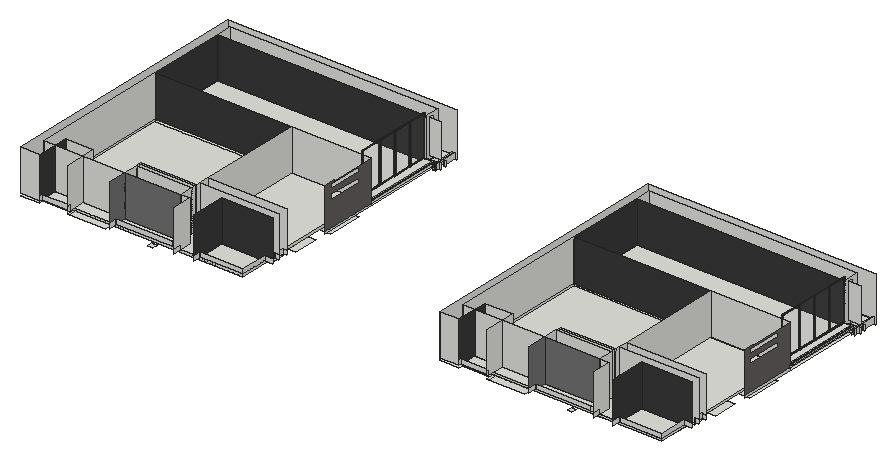
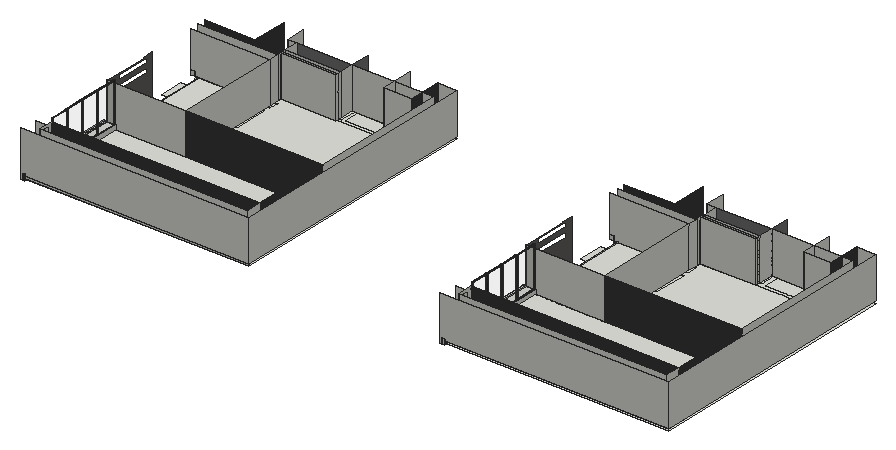
# SketchUp Ruby script. Lengths in inches.
U = 1.inch
M = Sketchup.active_model
def pt(a) = Geom::Point3d.new(a.map { |v| v * U })
def face(e, loops, mat)
  f = e.add_face(loops[0].map { |a| pt(a) })
  loops[1..].each { |l| e.add_face(l.map { |a| pt(a) }).erase! }
  f.material = f.back_material = mat if mat
  f
end
# faces: each face lists its corners as indices into pts; further lists are holes
def faces(e, pts, list, mat = nil) = list.each { |f| face(e, (f[0].is_a?(Array) ? f : [f]).map { |l| l.map { |i| pts[i] } }, mat) }
# xy, xz, yz: faces in a plane at the given z, y or x. An outline is a flat list of corners, or four numbers for a rectangle; further outlines are holes
def ring(l) = l.size == 4 ? [[l[0], l[1]], [l[2], l[1]], [l[2], l[3]], [l[0], l[3]]] : l.each_slice(2).to_a
def flat(e, list, mat, &to3) = list.each { |f| face(e, (f[0].is_a?(Array) ? f : [f]).map { |l| ring(l).map { |u, v| to3.(u, v) } }, mat) }
def xy(e, z, list, mat = nil) = flat(e, list, mat) { |x, y| [x, y, z] }
def xz(e, y, list, mat = nil) = flat(e, list, mat) { |x, z| [x, y, z] }
def yz(e, x, list, mat = nil) = flat(e, list, mat) { |y, z| [x, y, z] }
def lines(e, pts, list) = list.each { |a, b| e.add_line(pt(pts[a]), pt(pts[b])) }
# prism: a flat outline (further loops are holes) pulled along v
def prism(e, loops, v, mat = nil)
  f = face(e, loops, mat); d = Geom::Vector3d.new(v.map { |x| x * U })
  f.pushpull(f.normal.samedirection?(d) ? d.length : -d.length)
end
def box(e, o, s, mat = nil) = prism(e, [[o, [o[0] + s[0], o[1], o[2]], [o[0] + s[0], o[1] + s[1], o[2]], [o[0], o[1] + s[1], o[2]]]], [0, 0, s[2]], mat)
def at(x, y, z, deg = 0) = Geom::Transformation.translation(pt([x, y, z])) * Geom::Transformation.rotation(ORIGIN, Z_AXIS, deg.degrees)
def axes(o, x, y, z) = Geom::Transformation.new([*x, 0, *y, 0, *z, 0, *pt(o).to_a, 1])
def part(name) = M.definitions.add(name)
# library, detail: a bought-in or finely detailed component or shape, given as its bounding box
def library(name, o, s) = part(name).tap { |d| box(d.entities, o, s) }
def detail(e, o, s) = box(e.add_group.entities, o, s)
def put(e, d, t, mat = nil) = e.add_instance(d, t).tap { |i| i.material = mat if mat }
def group(e, t, mat = nil) = e.add_group.tap { |g| g.transformation = t; g.material = mat if mat }.entities
root = M.entities
M.materials.add("Glazing").color = [128, 128, 128]
M.materials["Glazing"].alpha = 0.05
M.materials.add("Powdercoating").color = [41, 44, 40]
M.materials.add("[Color M05]").color = [114, 114, 114]
M.materials.add("[Color M07]").color = [58, 58, 58]
M.materials.add("[Concrete Tile]").color = [165, 155, 133]
M.materials.add("[Stone Marble]").color = [99, 95, 94]
c1 = part("Group\#15")
xy(c1.entities,0,[[0,-55.94,0.71,45.94]])
xy(c1.entities,0.2,[[0,-55.94,0.47,45.94],[0.47,45.94,0.71,46.42]])
xy(c1.entities,2.36,[[0.47,-55.94,0.71,46.42]])
xz(c1.entities,-55.94,[[0,0,0.71,0,0.71,2.36,0.47,2.36,0.47,0.2,0,0.2]])
xz(c1.entities,45.94,[[0,0,0.71,0.2]])
xz(c1.entities,46.42,[[0.47,0.2,0.71,2.36]])
yz(c1.entities,0,[[-55.94,0,45.94,0.2]])
yz(c1.entities,0.47,[[-55.94,0.2,46.42,2.36]])
yz(c1.entities,0.71,[[-55.94,0,45.94,0,45.94,0.2,46.42,0.2,46.42,2.36,-55.94,2.36]])
c2 = part("Group\#7")
xy(c2.entities,0,[[0,-59.09,0.71,45.94]])
xy(c2.entities,0.2,[[0,-59.09,0.47,45.94],[0.47,45.94,0.71,46.42]])
xy(c2.entities,2.36,[[0.47,-59.09,0.71,46.42]])
xz(c2.entities,-59.09,[[0,0,0.71,0,0.71,2.36,0.47,2.36,0.47,0.2,0,0.2]])
xz(c2.entities,45.94,[[0,0,0.71,0.2]])
xz(c2.entities,46.42,[[0.47,0.2,0.71,2.36]])
yz(c2.entities,0,[[-59.09,0,45.94,0.2]])
yz(c2.entities,0.47,[[-59.09,0.2,46.42,2.36]])
yz(c2.entities,0.71,[[-59.09,0,45.94,0,45.94,0.2,46.42,0.2,46.42,2.36,-59.09,2.36]])
c3 = part("Group\#16")
prism(c3.entities,[[[0.47,-56.18,0.2],[0,-56.18,0.2],[0,-56.18,0],[0.71,-56.18,0],[0.71,-56.18,2.36],[0.47,-56.18,2.36]]],[0,28.68,0])
c4 = part("Group\#10")
box(c4.entities,[-0.73,0,0],[27.99,0.55,102.05])
c5 = part("Group\#18")
xy(c5.entities,0,[[0.47,-56.18,0.47,-55.47,0,-55.47,0,-28.21,1.18,-28.21,1.18,-56.18]])
xy(c5.entities,0.2,[[0.71,-56.18,1.18,-28.21],[0,-55.47,0.47,-28.21],[0.47,-28.21,0.71,-27.74]])
xy(c5.entities,2.36,[[0.47,-56.18,0.71,-27.74]])
xz(c5.entities,-56.18,[[0.47,0,1.18,0,1.18,0.2,0.71,0.2,0.71,2.36,0.47,2.36]])
xz(c5.entities,-55.47,[[0,0,0.47,0.2]])
xz(c5.entities,-28.21,[[0,0,1.18,0.2]])
xz(c5.entities,-27.74,[[0.47,0.2,0.71,2.36]])
yz(c5.entities,0,[[-55.47,0,-28.21,0.2]])
yz(c5.entities,0.47,[[-56.18,0,-55.47,0.2],[-56.18,0.2,-27.74,2.36]])
yz(c5.entities,0.71,[[-56.18,0.2,-27.74,2.36]])
yz(c5.entities,1.18,[[-56.18,0,-28.21,0.2]])
c6 = part("Group\#34")
xy(c6.entities,0,[[-20.45,0,7.76,1.22]])
xy(c6.entities,0.06,[[-20.39,0.06,7.7,1.22]])
xy(c6.entities,0.47,[[-19.98,0,7.28,0.06]])
xy(c6.entities,101.89,[[-19.98,0,7.28,0.06]])
xy(c6.entities,102.3,[[-20.39,0.06,7.7,1.22]])
xy(c6.entities,102.36,[[-20.45,0,7.76,1.22]])
xz(c6.entities,0,[[[-20.45,0,7.76,102.36],[-19.98,0.47,7.28,101.89]]])
xz(c6.entities,0.06,[[[-20.39,0.06,7.7,102.3],[-19.98,0.47,7.28,101.89]]])
xz(c6.entities,1.22,[[[-20.45,0,7.76,102.36],[-20.39,0.06,7.7,102.3]]])
yz(c6.entities,-20.45,[[0,0,1.22,102.36]])
yz(c6.entities,-20.39,[[0.06,0.06,1.22,102.3]])
yz(c6.entities,-19.98,[[0,0.47,0.06,101.89]])
yz(c6.entities,7.28,[[0,0.47,0.06,101.89]])
yz(c6.entities,7.7,[[0.06,0.06,1.22,102.3]])
yz(c6.entities,7.76,[[0,0,1.22,102.36]])
c7 = part("Group\#6")
put(c7.entities,c1,axes([27.97,0,7.875],[1,0,0],[0,0,-1],[0,1,0]),"Powdercoating")
put(c7.entities,c2,axes([0.71,0,6.8],[-1,0,0],[0,0,-0.97687],[0,1,0]),"Powdercoating")
put(c7.entities,c3,axes([-27.5,0,-38.07],[0,0,-1],[-1,0,0],[0,1,0]),"Powdercoating")
put(c7.entities,c4,at(1.12,0.35,-38.39),"Glazing")
put(c7.entities,c5,axes([-27.5,0,63.35],[0,0,1],[-1,0,0],[0,1,0]),"Powdercoating")
put(c7.entities,c6,at(20.6875,1.0625,-38.54),"Powdercoating")
c8 = part("Sliding door assembly")
put(c8.entities,c7,at(-1.18,4.5,38.86))
g1 = group(c8.entities,at(84.74,4.5,38.86))
put(g1,c1,axes([-27.97,0,7.875],[-1,0,0],[0,0,-1],[0,1,0]),"Powdercoating")
put(g1,c2,axes([-0.71,0,6.8],[1,0,0],[0,0,-0.97687],[0,1,0]),"Powdercoating")
put(g1,c3,axes([27.5,0,-38.07],[0,0,-1],[1,0,0],[0,1,0]),"Powdercoating")
put(g1,c4,axes([-1.12,0.35,-38.39],[-1,0,0],[0,1,0],[0,0,1]),"Glazing")
put(g1,c5,axes([27.5,0,63.35],[0,0,1],[1,0,0],[0,1,0]),"Powdercoating")
put(g1,c6,axes([-20.6875,1.0625,-38.54],[-1,0,0],[0,1,0],[0,0,1]),"Powdercoating")
g2 = group(c8.entities,at(56.0625,4.5,38.86))
put(g2,c1,axes([-27.97,0,7.875],[-1,0,0],[0,0,-1],[0,1,0]),"Powdercoating")
put(g2,c3,axes([27.5,0,-38.07],[0,0,-1],[1,0,0],[0,1,0]),"Powdercoating")
put(g2,c4,axes([-1.12,0.35,-38.39],[-1,0,0],[0,1,0],[0,0,1]),"Glazing")
put(g2,c5,axes([27.5,0,63.35],[0,0,1],[1,0,0],[0,1,0]),"Powdercoating")
put(g2,c6,axes([-20.6875,1.0625,-38.54],[-1,0,0],[0,1,0],[0,0,1]),"Powdercoating")
g3 = group(g2,at(-0.71,0,6.8),"Powdercoating")
xy(g3,-45.34,[[0.47,0.2,0.71,2.36]])
xy(g3,-44.88,[[0,0,0.71,0.2]])
xy(g3,57.73,[[0,0,0.71,0,0.71,2.36,0.47,2.36,0.47,0.2,0,0.2]])
xz(g3,0,[[0,-44.88,0.71,57.73]])
xz(g3,0.2,[[0.47,-45.34,0.71,-44.88],[0,-44.88,0.47,57.73]])
xz(g3,2.36,[[0.47,-45.34,0.71,57.73]])
yz(g3,0,[[0,-44.88,0.2,57.73]])
yz(g3,0.47,[[0.2,-45.34,2.36,57.73]])
yz(g3,0.71,[[0.2,-45.34,2.36,-45.34,2.36,57.73,0,57.73,0,-44.88,0.2,-44.88]])
put(c8.entities,c7,axes([-33.94,4.5,38.86],[1.14218,0,0],[0,1,0],[0,0,1]))
c9 = part("sliding door")
put(c9.entities,c8,at(0,-4.5,-0.08))
xy(root,117.41,[[671.25,2113.57,913.875,2213.62],[1889.4375,2113.57,2132.0625,2213.62]])
xy(root,126,[[262.875,1799.9375,262.875,2554.375,913.875,2554.375,913.875,2483.21,890.875,2483.21,890.875,2531.375,285.875,2531.375,285.875,1822.9375,319.53,1822.9375,319.53,1799.9375],[399.88,1799.9375,406.68,1822.9375],[406.68,1799.9375,511.23,1822.9375],[634.11,1799.9375,647.8,1814.92],[1481.0625,1799.9375,1481.0625,2554.375,2132.0625,2554.375,2132.0625,2483.21,2109.0625,2483.21,2109.0625,2531.375,1504.0625,2531.375,1504.0625,1822.9375,1537.72,1822.9375,1537.72,1799.9375],
  [1618.07,1799.9375,1624.87,1822.9375],[1624.87,1799.9375,1729.42,1822.9375],[1852.3,1799.9375,1865.99,1814.92],[319.53,1811.4375,399.88,1822.9375],[1537.72,1811.4375,1618.07,1822.9375],
  [285.875,1822.9375,319.53,1834.0625],[319.53,1822.9375,399.88,1834.0625],[399.88,1822.9375,406.68,1834.0625],[406.68,1822.9375,511.23,1834.0625],[511.23,1822.9375,521.59,1834.0625],
  [521.59,1822.9375,634.11,1834.0625],[634.11,1822.9375,709.87,1834.0625],[709.87,1822.9375,767.19,1834.0625],[767.19,1822.9375,817,1834.0625],[817,1822.9375,890.875,1834.0625],
  [1504.0625,1822.9375,1537.72,1834.0625],[1537.72,1822.9375,1618.07,1834.0625],[1618.07,1822.9375,1624.87,1834.0625],[1624.87,1822.9375,1729.42,1834.0625],[1729.42,1822.9375,1739.78,1834.0625],
  [1739.78,1822.9375,1852.3,1834.0625],[1852.3,1822.9375,1928.05,1834.0625],[1928.05,1822.9375,1985.38,1834.0625],[1985.38,1822.9375,2035.1875,1834.0625],[2035.1875,1822.9375,2109.0625,1834.0625],
  [285.875,1834.0625,319.53,1834.0625,319.53,1893.25,399.88,1893.25,399.88,1834.0625,406.68,1834.0625,406.68,1893.25,511.23,1893.25,511.23,1834.0625,521.59,1834.0625,521.59,1893.25,709.87,1893.25,709.87,1834.0625,767.19,1834.0625,767.19,1902.66,285.875,1902.66],[319.53,1834.0625,399.88,1893.25],[406.68,1834.0625,511.23,1893.25],[521.59,1834.0625,634.11,1893.25],[634.11,1834.0625,709.87,1893.25],
  [767.19,1834.0625,817,1902.66],[817,1834.0625,890.875,1902.66],[1504.0625,1834.0625,1537.72,1834.0625,1537.72,1893.25,1618.07,1893.25,1618.07,1834.0625,1624.87,1834.0625,1624.87,1893.25,1729.42,1893.25,1729.42,1834.0625,1739.78,1834.0625,1739.78,1893.25,1928.05,1893.25,1928.05,1834.0625,1985.38,1834.0625,1985.38,1902.66,1504.0625,1902.66],[1537.72,1834.0625,1618.07,1893.25],[1624.87,1834.0625,1729.42,1893.25],
  [1739.78,1834.0625,1852.3,1893.25],[1852.3,1834.0625,1928.05,1893.25],[1985.38,1834.0625,2035.1875,1902.66],[2035.1875,1834.0625,2109.0625,1902.66],[285.875,1902.66,817,1902.66,817,1926.07,683.6875,1926.07,683.6875,1953.7,817,1953.7,817,1970.91,683.6875,1970.91,683.6875,2070.28,890.875,2070.28,890.875,2257.8125,285.875,2257.8125],
  [817,1902.66,890.875,1926.07],[1504.0625,1902.66,2035.1875,1902.66,2035.1875,1926.07,1901.875,1926.07,1901.875,1953.7,2035.1875,1953.7,2035.1875,1970.91,1901.875,1970.91,1901.875,2070.28,2109.0625,2070.28,2109.0625,2257.8125,1504.0625,2257.8125],[2035.1875,1902.66,2109.0625,1926.07],[683.6875,1926.07,817,1953.7],[817,1926.07,890.875,1953.7],
  [890.875,1926.07,902.375,1953.7],[1901.875,1926.07,2035.1875,1953.7],[1901.875,1926.07,2035.1875,1953.7],[2035.1875,1926.07,2109.0625,1953.7],[2109.0625,1926.07,2120.5625,1953.7],
  [817,1953.7,890.875,1970.91],[2035.1875,1953.7,2109.0625,1970.91],[683.6875,1970.91,890.875,2070.28],[1901.875,1970.91,2109.0625,2070.28],[890.875,1987.85,913.875,2059.15],
  [2109.0625,1987.85,2132.0625,2059.15],[285.875,2257.8125,890.875,2485.84],[890.875,2257.8125,913.875,2483.21],[1504.0625,2257.8125,2109.0625,2485.84],[2109.0625,2257.8125,2132.0625,2483.21]])
xy(root,132,[[262.875,1799.9375,262.875,2554.375,913.875,2554.375,913.875,2483.21,890.875,2483.21,890.875,2531.375,285.875,2531.375,285.875,1822.9375,319.53,1822.9375,319.53,1799.9375],[1481.0625,1799.9375,1481.0625,2554.375,2132.0625,2554.375,2132.0625,2483.21,2109.0625,2483.21,2109.0625,2531.375,1504.0625,2531.375,1504.0625,1822.9375,1537.72,1822.9375,1537.72,1799.9375],[319.53,1807.625,399.88,1822.9375],[1537.72,1807.625,1618.07,1822.9375],[285.875,1822.9375,319.53,1855.75],
  [319.53,1822.9375,399.88,1855.75],[399.88,1822.9375,523.04,1855.75],[523.04,1822.9375,683.6875,1855.75],[683.6875,1822.9375,709.87,1855.75],[709.87,1822.9375,709.87,1855.75,683.6875,1855.75,683.6875,1926.07,890.875,1926.07,890.875,1902.66,767.19,1902.66,767.19,1822.9375],
  [767.19,1822.9375,890.875,1902.66],[1504.0625,1822.9375,1537.72,1855.75],[1537.72,1822.9375,1618.07,1855.75],[1618.07,1822.9375,1741.23,1855.75],[1741.23,1822.9375,1901.875,1855.75],
  [1901.875,1822.9375,1928.05,1855.75],[1928.05,1822.9375,1928.05,1855.75,1901.875,1855.75,1901.875,1926.07,2109.0625,1926.07,2109.0625,1902.66,1985.38,1902.66,1985.38,1822.9375],[1985.38,1822.9375,2109.0625,1902.66],[319.53,1855.75,399.88,1893.25],[523.04,1855.75,683.6875,1897.5625],
  [1537.72,1855.75,1618.07,1893.25],[1741.23,1855.75,1901.875,1897.5625],[523.04,1897.5625,683.6875,1906.6875],[1741.23,1897.5625,1901.875,1906.6875],[523.04,1906.6875,683.6875,1913.4375],
  [1741.23,1906.6875,1901.875,1913.4375],[683.6875,1926.07,890.875,1953.7],[890.875,1926.07,902.375,1953.7],[1901.875,1926.07,2109.0625,1953.7],[2109.0625,1926.07,2120.5625,1953.7],
  [683.6875,1953.7,890.875,2258.18],[1901.875,1953.7,2109.0625,2258.18],[285.875,2258.18,886.75,2258.18,886.75,2483.21,890.875,2483.21,890.875,2486.82,285.875,2486.82],[886.75,2258.18,890.875,2483.21],[890.875,2258.18,913.875,2483.21],
  [1504.0625,2258.18,2104.9375,2258.18,2104.9375,2483.21,2109.0625,2483.21,2109.0625,2486.82,1504.0625,2486.82],[2104.9375,2258.18,2109.0625,2483.21],[2109.0625,2258.18,2132.0625,2483.21]])
xy(root,143.875,[[913.875,2257.8125,921.125,2258.18],[2132.0625,2257.8125,2139.3125,2258.18],[886.75,2258.18,913.875,2483.21],[913.875,2258.18,921.125,2483.21],[2104.9375,2258.18,2132.0625,2483.21],
  [2132.0625,2258.18,2139.3125,2483.21],[913.875,2483.21,921.125,2486.82],[2132.0625,2483.21,2139.3125,2486.82]])
xy(root,144.25,[[913.875,2257.8125,921.125,2258.18],[2132.0625,2257.8125,2139.3125,2258.18]])
xz(root,1799.9375,[[262.875,132,319.53,252],[1481.0625,132,1537.72,252]])
xz(root,1799.9375,[[521.59,132,523.04,252],[1739.78,132,1741.23,252]],"[Concrete Tile]")
xz(root,1807.625,[[319.53,132,399.88,145.375],[1537.72,132,1618.07,145.375]])
xz(root,1814.92,[[634.11,124.32,647.8,126],[1852.3,124.32,1865.99,126]])
xz(root,1822.9375,[[285.875,126,890.875,132],[1504.0625,126,2109.0625,132],[523.04,132,683.6875,145.375],[683.6875,132,709.87,145.375],[767.19,132,890.875,145.375],
  [1741.23,132,1901.875,145.375],[1901.875,132,1928.05,145.375],[1985.38,132,2109.0625,145.375]])
xz(root,1855.75,[[285.875,132,523.04,252],[683.6875,132,709.87,252],[1504.0625,132,1741.23,252],[1901.875,132,1928.05,252]])
xz(root,1855.75,[[523.04,132,683.6875,252],[1741.23,132,1901.875,252]],"[Color M05]")
xz(root,1893.25,[[319.53,132,399.88,252],[1537.72,132,1618.07,252]])
xz(root,1897.5625,[[523.04,132,683.6875,252],[1741.23,132,1901.875,252]])
xz(root,1902.66,[[890.875,132,913.875,145.375],[2109.0625,132,2132.0625,145.375]])
xz(root,1902.66,[[767.19,132,890.875,132,890.875,147.125,913.875,147.125,913.875,252,767.19,252],[1985.38,132,2109.0625,132,2109.0625,147.125,2132.0625,147.125,2132.0625,252,1985.38,252]],"[Color M07]")
xz(root,1906.6875,[[523.04,132,683.6875,252],[1741.23,132,1901.875,252]])
xz(root,1913.4375,[[523.04,132,683.6875,252],[1741.23,132,1901.875,252]])
xz(root,1926.07,[[683.6875,132,683.6875,252,913.875,252,913.875,145.375,902.375,145.375,902.375,132],[902.375,132,913.875,145.375],[1901.875,132,1901.875,252,2132.0625,252,2132.0625,145.375,2120.5625,145.375,2120.5625,132],[2120.5625,132,2132.0625,145.375]])
xz(root,1953.7,[[683.6875,132,902.375,132,902.375,145.375,913.875,145.375,913.875,252,683.6875,252],[902.375,132,913.875,145.375],[1901.875,132,2120.5625,132,2120.5625,145.375,2132.0625,145.375,2132.0625,252,1901.875,252],[2120.5625,132,2132.0625,145.375]])
xz(root,2257.8125,[[913.875,143.875,921.125,144.25],[2132.0625,143.875,2139.3125,144.25]])
xz(root,2258.18,[[683.6875,132,683.6875,252,913.875,252,913.875,143.875,886.75,143.875,886.75,132],[886.75,132,913.875,143.875],[1901.875,132,1901.875,252,2132.0625,252,2132.0625,143.875,2104.9375,143.875,2104.9375,132],[2104.9375,132,2132.0625,143.875],[913.875,143.875,921.125,144.25],
  [2132.0625,143.875,2139.3125,144.25],[913.875,144.25,921.125,145.375],[2132.0625,144.25,2139.3125,145.375]])
xz(root,2258.18,[[285.875,132,683.6875,252],[1504.0625,132,1901.875,252]],"[Color M07]")
xz(root,2483.21,[[886.75,132,890.875,136.875],[2104.9375,132,2109.0625,136.875],[886.75,136.875,890.875,143.875],[2104.9375,136.875,2109.0625,143.875],[913.875,143.875,921.125,145.375],
  [2132.0625,143.875,2139.3125,145.375]])
xz(root,2483.21,[[890.875,132,913.875,136.875],[2109.0625,132,2132.0625,136.875],[890.875,136.875,913.875,143.875],[2109.0625,136.875,2132.0625,143.875]],"[Color M07]")
xz(root,2486.82,[[913.875,120.4375,921.125,136.875],[2132.0625,120.4375,2139.3125,136.875],[913.875,136.875,921.125,143.875],[2132.0625,136.875,2139.3125,143.875]])
xz(root,2486.82,[[285.875,132,890.875,252],[1504.0625,132,2109.0625,252]],"[Color M07]")
xz(root,2497.47,[[921.125,120.4375,927.0625,136.875],[2139.3125,120.4375,2145.25,136.875],[927.0625,143.875,927.0625,145.375,890.875,145.375,890.875,245.15,927.75,245.15,927.75,143.875],[2145.25,143.875,2145.25,145.375,2109.0625,145.375,2109.0625,245.15,2145.9375,245.15,2145.9375,143.875]])
xz(root,2514.84,[[921.125,120.4375,927.0625,136.875],[2139.3125,120.4375,2145.25,136.875]])
xz(root,2531.375,[[285.875,126,890.875,132],[1504.0625,126,2109.0625,132],[285.875,132,890.875,252],[1504.0625,132,2109.0625,252]])
xz(root,2554.375,[[921.125,120.4375,921.125,136.875,913.875,136.875,913.875,132,262.875,132,262.875,252,927.75,252,927.75,120.4375],[913.875,120.4375,921.125,136.875],[2139.3125,120.4375,2139.3125,136.875,2132.0625,136.875,2132.0625,132,1481.0625,132,1481.0625,252,2145.9375,252,2145.9375,120.4375],[2132.0625,120.4375,2139.3125,136.875],[1481.0625,126,2132.0625,132]])
yz(root,262.875,[[1799.9375,132,2554.375,252]])
yz(root,285.875,[[1822.9375,126,2531.375,132],[1855.75,132,2258.18,252],[2486.82,132,2531.375,252]])
yz(root,285.875,[[2258.18,132,2486.82,252]],"[Color M07]")
yz(root,319.53,[[1799.9375,132,1807.625,145.375]])
yz(root,319.53,[[1807.625,132,1893.25,132,1893.25,252,1799.9375,252,1799.9375,145.375,1807.625,145.375]],"[Color M07]")
yz(root,399.88,[[1799.9375,132,1807.625,145.375],[1807.625,132,1807.625,145.375,1799.9375,145.375,1799.9375,252,1893.25,252,1893.25,132]])
yz(root,523.04,[[1799.9375,132,1822.9375,145.375],[1855.75,132,1897.5625,252],[1897.5625,132,1906.6875,252],[1906.6875,132,1913.4375,252]])
yz(root,523.04,[[1822.9375,132,1855.75,132,1855.75,252,1799.9375,252,1799.9375,145.375,1822.9375,145.375]],"[Color M05]")
yz(root,683.6875,[[1855.75,132,1897.5625,252],[1897.5625,132,1906.6875,252],[1906.6875,132,1913.4375,252],[1913.4375,132,1926.07,252],[1926.07,132,1953.7,252],
  [1953.7,132,2258.18,252]])
yz(root,709.87,[[1799.9375,132,1822.9375,145.375],[1822.9375,132,1822.9375,145.375,1799.9375,145.375,1799.9375,252,1855.75,252,1855.75,132]])
yz(root,767.19,[[1799.9375,132,1822.9375,145.375]])
yz(root,767.19,[[1822.9375,132,1902.66,132,1902.66,252,1799.9375,252,1799.9375,147.125,1822.9375,147.125]],"[Color M07]")
yz(root,886.75,[[2258.18,132,2483.21,143.875]])
yz(root,890.875,[[1822.9375,126,2531.375,132],[1822.9375,132,1902.66,145.375],[2483.21,132,2486.82,252],[[2486.82,132,2531.375,252],[2497.47,145.375,2514.84,245.15]]])
yz(root,902.375,[[1926.07,132,1953.7,145.375]])
yz(root,913.875,[[2483.21,120.4375,2486.82,126],[2486.82,120.4375,2554.375,126],[2093.65,126,2257.8125,132],[2486.82,126,2554.375,132],[2257.8125,132,2258.18,143.875],
  [2258.18,132,2483.21,143.875],[2483.21,132,2486.82,136.875],[2486.82,132,2554.375,136.875],[2483.21,136.875,2486.82,143.875],[2257.8125,143.875,2258.18,144.25],
  [2258.18,143.875,2483.21,145.375]])
yz(root,913.875,[[[2093.65,132,2257.8125,132,2257.8125,144.25,2258.18,144.25,2258.18,248.9375,2124.51,248.9375,2124.51,252,2093.65,252],[2113.57,206.6875,2213.62,220.18],[2113.57,234.11,2213.62,246.61]]],"[Stone Marble]")
yz(root,921.125,[[2484.2,120.4375,2486.82,136.875],[2486.82,120.4375,2497.47,136.875],[2514.84,120.4375,2554.375,136.875],[2484.2,136.875,2486.82,143.875],[2257.8125,143.875,2258.18,144.25],
  [2258.18,143.875,2483.21,145.375]])
yz(root,1481.0625,[[1799.9375,132,2554.375,252]])
yz(root,1504.0625,[[1822.9375,126,2531.375,132],[1855.75,132,2258.18,252],[2486.82,132,2531.375,252]])
yz(root,1504.0625,[[2258.18,132,2486.82,252]],"[Color M07]")
yz(root,1537.72,[[1799.9375,132,1807.625,145.375]])
yz(root,1537.72,[[1807.625,132,1893.25,132,1893.25,252,1799.9375,252,1799.9375,145.375,1807.625,145.375]],"[Color M07]")
yz(root,1618.07,[[1799.9375,132,1807.625,145.375],[1807.625,132,1807.625,145.375,1799.9375,145.375,1799.9375,252,1893.25,252,1893.25,132]])
yz(root,1741.23,[[1799.9375,132,1822.9375,145.375],[1855.75,132,1897.5625,252],[1897.5625,132,1906.6875,252],[1906.6875,132,1913.4375,252]])
yz(root,1741.23,[[1822.9375,132,1855.75,132,1855.75,252,1799.9375,252,1799.9375,145.375,1822.9375,145.375]],"[Color M05]")
yz(root,1901.875,[[1855.75,132,1897.5625,252],[1897.5625,132,1906.6875,252],[1906.6875,132,1913.4375,252],[1913.4375,132,1926.07,252],[1926.07,132,1953.7,252],
  [1926.07,132,1953.7,252],[1953.7,132,2258.18,252]])
yz(root,1928.05,[[1799.9375,132,1822.9375,145.375],[1822.9375,132,1822.9375,145.375,1799.9375,145.375,1799.9375,252,1855.75,252,1855.75,132]])
yz(root,1985.38,[[1799.9375,132,1822.9375,145.375]])
yz(root,1985.38,[[1822.9375,132,1902.66,132,1902.66,252,1799.9375,252,1799.9375,147.125,1822.9375,147.125]],"[Color M07]")
yz(root,2104.9375,[[2258.18,132,2483.21,143.875]])
yz(root,2109.0625,[[1822.9375,126,2531.375,132],[1822.9375,132,1902.66,145.375],[2483.21,132,2486.82,252],[[2486.82,132,2531.375,252],[2497.47,145.375,2514.84,245.15]]])
yz(root,2120.5625,[[1926.07,132,1953.7,145.375]])
yz(root,2132.0625,[[2483.21,120.4375,2486.82,126],[2486.82,120.4375,2554.375,126],[2093.65,126,2257.8125,132],[2486.82,126,2554.375,132],[2257.8125,132,2258.18,143.875],
  [2258.18,132,2483.21,143.875],[2483.21,132,2486.82,136.875],[2486.82,132,2554.375,136.875],[2483.21,136.875,2486.82,143.875],[2257.8125,143.875,2258.18,144.25],
  [2258.18,143.875,2483.21,145.375]])
yz(root,2132.0625,[[[2093.65,132,2257.8125,132,2257.8125,144.25,2258.18,144.25,2258.18,248.9375,2124.51,248.9375,2124.51,252,2093.65,252],[2113.57,206.6875,2213.62,220.18],[2113.57,234.11,2213.62,246.61]]],"[Stone Marble]")
yz(root,2139.3125,[[2484.2,120.4375,2486.82,136.875],[2486.82,120.4375,2497.47,136.875],[2514.84,120.4375,2554.375,136.875],[2484.2,136.875,2486.82,143.875],[2257.8125,143.875,2258.18,144.25],
  [2258.18,143.875,2483.21,145.375]])
p = [[2132.0625,2485.84,120.4375],[2139.3125,2485.84,120.4375],[913.875,2485.84,120.4375],[921.125,2485.84,120.4375]]
lines(root,p,[[0,1],[2,3]])
put(root,c9,axes([2109.0625,2323.22,143.875],[0,1.90384,0],[-1,0,0],[0,0,1.13691]),"[Color M07]")
put(root,c9,axes([890.875,2323.22,143.875],[0,1.90384,0],[-1,0,0],[0,0,1.13691]),"[Color M07]")
